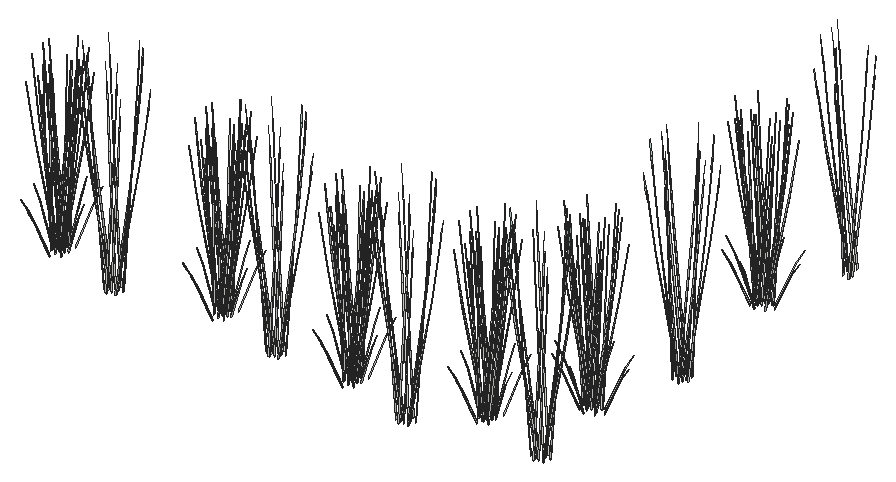
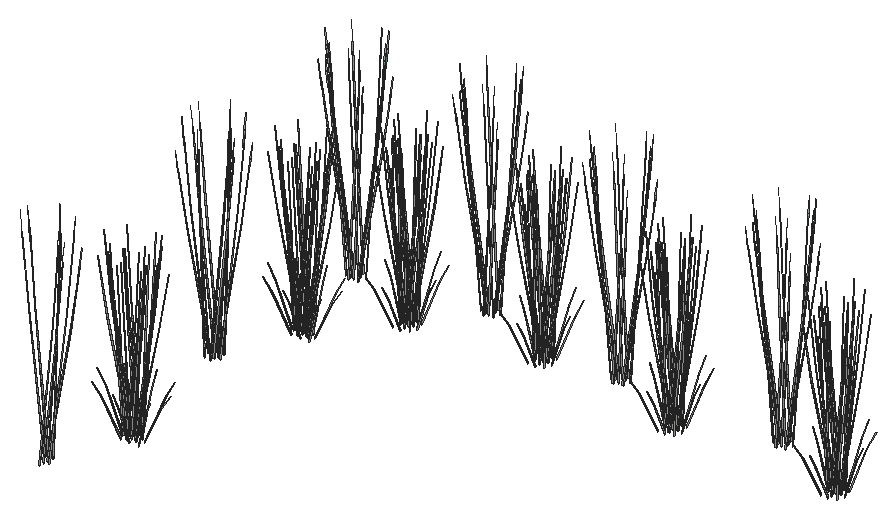
# SketchUp Ruby script. Lengths in inches.
U = 1.inch
M = Sketchup.active_model
def pt(a) = Geom::Point3d.new(a.map { |v| v * U })
def face(e, loops, mat)
  f = e.add_face(loops[0].map { |a| pt(a) })
  loops[1..].each { |l| e.add_face(l.map { |a| pt(a) }).erase! }
  f.material = f.back_material = mat if mat
  f
end
# faces: each face lists its corners as indices into pts; further lists are holes
def faces(e, pts, list, mat = nil) = list.each { |f| face(e, (f[0].is_a?(Array) ? f : [f]).map { |l| l.map { |i| pts[i] } }, mat) }
# xy, xz, yz: faces in a plane at the given z, y or x. An outline is a flat list of corners, or four numbers for a rectangle; further outlines are holes
def ring(l) = l.size == 4 ? [[l[0], l[1]], [l[2], l[1]], [l[2], l[3]], [l[0], l[3]]] : l.each_slice(2).to_a
def flat(e, list, mat, &to3) = list.each { |f| face(e, (f[0].is_a?(Array) ? f : [f]).map { |l| ring(l).map { |u, v| to3.(u, v) } }, mat) }
def xy(e, z, list, mat = nil) = flat(e, list, mat) { |x, y| [x, y, z] }
def xz(e, y, list, mat = nil) = flat(e, list, mat) { |x, z| [x, y, z] }
def yz(e, x, list, mat = nil) = flat(e, list, mat) { |y, z| [x, y, z] }
def lines(e, pts, list) = list.each { |a, b| e.add_line(pt(pts[a]), pt(pts[b])) }
# prism: a flat outline (further loops are holes) pulled along v
def prism(e, loops, v, mat = nil)
  f = face(e, loops, mat); d = Geom::Vector3d.new(v.map { |x| x * U })
  f.pushpull(f.normal.samedirection?(d) ? d.length : -d.length)
end
def box(e, o, s, mat = nil) = prism(e, [[o, [o[0] + s[0], o[1], o[2]], [o[0] + s[0], o[1] + s[1], o[2]], [o[0], o[1] + s[1], o[2]]]], [0, 0, s[2]], mat)
def at(x, y, z, deg = 0) = Geom::Transformation.translation(pt([x, y, z])) * Geom::Transformation.rotation(ORIGIN, Z_AXIS, deg.degrees)
def axes(o, x, y, z) = Geom::Transformation.new([*x, 0, *y, 0, *z, 0, *pt(o).to_a, 1])
def part(name) = M.definitions.add(name)
# library, detail: a bought-in or finely detailed component or shape, given as its bounding box
def library(name, o, s) = part(name).tap { |d| box(d.entities, o, s) }
def detail(e, o, s) = box(e.add_group.entities, o, s)
def put(e, d, t, mat = nil) = e.add_instance(d, t).tap { |i| i.material = mat if mat }
def group(e, t, mat = nil) = e.add_group.tap { |g| g.transformation = t; g.material = mat if mat }.entities
root = M.entities
M.materials.add("LightPink_Translucent").color = [175, 214, 192]
M.materials["LightPink_Translucent"].alpha = 0.75
c1 = part("blade")
p = [[2.15,0.21,22],[0,0.17,0],[0.09,0.45,0],[2.18,0.31,22],[2.29,0.31,22],[0.38,0.45,0],
  [2.48,0.24,33],[2.49,0.24,33],[2.48,0.22,33]]
faces(c1.entities,p,[[0,1,2,3],[4,5,2,3],[6,3,4,7],[8,0,3,6]])
c2 = part("seeds")
p = [[0.3,-0.1,1.38],[-0.01,-0.03,1.59],[-0.01,-0.03,0.03],[0.14,-0.07,-0.07],[0.29,-0.03,3],[0.15,0.01,3.11]]
faces(c2.entities,p,[[0,1,2,3],[1,0,4,5]],"LightPink_Translucent")
c3 = part("blade with seeds")
put(c3.entities,c1,at(0,0,0))
put(c3.entities,c2,axes([2.4,0.25,30.99],[1.5799,-0.05474,1.17369],[-0.12525,1.92788,0.29478],[-0.07173,-0.02425,1.56792]))
c4 = part("blade with seeds\#1")
put(c4.entities,c1,at(0,0,0))
put(root,c3,axes([462.53,231.19,139.17],[-0.19628,-0.45667,-0.6355],[0.5654,-0.16447,-0.16679],[-0.02169,-0.15464,1.40276]))
put(root,c3,axes([461.38,231.125,139.1],[0,-0.44533,-0.45182],[0.53472,0,0],[0,-0.10143,1.43328]))
put(root,c3,axes([462.86,229.81,139.1],[0.44731,-0.22267,-0.45182],[0.26736,0.39927,0],[0.10188,-0.05071,1.43328]))
put(root,c3,axes([463.39,230.72,139.14],[0.32192,-0.33473,-0.56741],[0.39991,0.30352,-0.14892],[0.129,-0.0835,1.25246]))
put(root,c3,axes([462.61,232.04,139.14],[-0.49717,-0.07301,-0.56741],[0.10491,-0.45037,-0.14892],[-0.14837,-0.05457,1.25246]))
put(root,c3,axes([461.96,232.89,139.1],[-0.44731,-0.22267,-0.45182],[0.26736,-0.39927,0],[-0.10188,-0.05071,1.43328]))
put(root,c3,axes([464.93,230.26,139.1],[0.44731,0.22267,-0.45182],[-0.26736,0.39927,0],[0.10188,0.05071,1.43328]))
put(root,c3,axes([464.28,231.11,139.14],[0.49717,0.07301,-0.56741],[-0.10491,0.45037,-0.14892],[0.14837,0.05457,1.25246]))
put(root,c4,axes([445.51,235.44,138.04],[-0.05785,0.02598,1.44662],[-0.33839,-0.1802,-0.221],[-0.00487,-0.18177,0.24641]))
put(root,c3,axes([390.05,236.01,139.08],[-0.19628,-0.45667,-0.6355],[0.5654,-0.16447,-0.16679],[-0.02169,-0.15464,1.40276]))
put(root,c3,axes([428.25,236.01,139.08],[-0.19628,-0.45667,-0.6355],[0.5654,-0.16447,-0.16679],[-0.02169,-0.15464,1.40276]))
put(root,c3,axes([490.26,236.01,139.08],[-0.19628,-0.45667,-0.6355],[0.5654,-0.16447,-0.16679],[-0.02169,-0.15464,1.40276]))
put(root,c3,axes([388.9,235.94,139.01],[0,-0.44533,-0.45182],[0.53472,0,0],[0,-0.10143,1.43328]))
put(root,c3,axes([427.09,235.94,139.01],[0,-0.44533,-0.45182],[0.53472,0,0],[0,-0.10143,1.43328]))
put(root,c3,axes([489.1,235.94,139.01],[0,-0.44533,-0.45182],[0.53472,0,0],[0,-0.10143,1.43328]))
put(root,c3,axes([390.38,234.625,139.01],[0.44731,-0.22267,-0.45182],[0.26736,0.39927,0],[0.10188,-0.05071,1.43328]))
put(root,c3,axes([428.58,234.625,139.01],[0.44731,-0.22267,-0.45182],[0.26736,0.39927,0],[0.10188,-0.05071,1.43328]))
put(root,c3,axes([490.59,234.625,139.01],[0.44731,-0.22267,-0.45182],[0.26736,0.39927,0],[0.10188,-0.05071,1.43328]))
put(root,c3,axes([390.91,235.54,139.04],[0.32192,-0.33473,-0.56741],[0.39991,0.30352,-0.14892],[0.129,-0.0835,1.25246]))
put(root,c3,axes([429.11,235.54,139.04],[0.32192,-0.33473,-0.56741],[0.39991,0.30352,-0.14892],[0.129,-0.0835,1.25246]))
put(root,c3,axes([491.12,235.54,139.04],[0.32192,-0.33473,-0.56741],[0.39991,0.30352,-0.14892],[0.129,-0.0835,1.25246]))
put(root,c4,axes([445.2,237.41,138.5],[0.06247,-0.51713,-0.51151],[0.38535,0.10913,-0.13425],[0.04669,-0.15433,1.12907]))
put(root,c4,axes([447.18,236.76,138.04],[-0.05501,-0.03622,1.44662],[-0.16202,-0.45599,-0.221],[0.08385,-0.13824,0.24641]))
put(root,c3,axes([463.5,232.43,139.14],[-0.32192,0.33473,-0.56741],[-0.39991,-0.30352,-0.14892],[-0.129,0.0835,1.25246]))
put(root,c4,axes([444.47,236.73,138.47],[0.19052,-0.46527,-0.40731],[0.34163,0.2781,0],[0.04339,-0.10597,1.29208]))
put(root,c3,axes([464.03,233.34,139.1],[-0.44731,0.22267,-0.45182],[-0.26736,-0.39927,0],[-0.10188,0.05071,1.43328]))
put(root,c3,axes([465.51,232.03,139.1],[0,0.44533,-0.45182],[-0.53472,0,0],[0,0.10143,1.43328]))
put(root,c4,axes([444.07,236.5,138.04],[-0.03002,0.07441,1.44662],[-0.33536,0.19113,-0.221],[-0.09101,-0.12893,0.24641]))
put(root,c3,axes([464.33,231.97,139.17],[0.17525,0.40774,-0.62983],[-0.50482,0.14685,-0.1653],[0.01937,0.13807,1.39023]))
put(root,c4,axes([444.61,236.86,138.48],[0.33202,-0.11678,-0.25413],[0.09428,0.4638,0.25413],[0.03829,-0.0935,1.14007]))
put(root,c4,axes([444.87,238.33,138.5],[-0.2864,-0.33485,-0.51151],[0.2597,-0.41596,-0.13425],[-0.07144,-0.13418,1.12907]))
put(root,c3,axes([390.13,236.86,139.04],[-0.49717,-0.07301,-0.56741],[0.10491,-0.45037,-0.14892],[-0.14837,-0.05457,1.25246]))
put(root,c3,axes([428.32,236.86,139.04],[-0.49717,-0.07301,-0.56741],[0.10491,-0.45037,-0.14892],[-0.14837,-0.05457,1.25246]))
put(root,c3,axes([490.34,236.86,139.04],[-0.49717,-0.07301,-0.56741],[0.10491,-0.45037,-0.14892],[-0.14837,-0.05457,1.25246]))
put(root,c4,axes([445.32,237.68,138.625],[0.31983,-0.29864,-0.36702],[0.22522,0.45236,0.17663],[0.03957,-0.09664,1.17838]))
put(root,c4,axes([445.98,236.13,138.47],[0.38104,0,-0.40731],[0,0.5562,0],[0.08679,0,1.29208]))
put(root,c3,axes([389.48,237.71,139.01],[-0.44731,-0.22267,-0.45182],[0.26736,-0.39927,0],[-0.10188,-0.05071,1.43328]))
put(root,c3,axes([427.67,237.71,139.01],[-0.44731,-0.22267,-0.45182],[0.26736,-0.39927,0],[-0.10188,-0.05071,1.43328]))
put(root,c3,axes([489.68,237.71,139.01],[-0.44731,-0.22267,-0.45182],[0.26736,-0.39927,0],[-0.10188,-0.05071,1.43328]))
put(root,c3,axes([392.45,235.08,139.01],[0.44731,0.22267,-0.45182],[-0.26736,0.39927,0],[0.10188,0.05071,1.43328]))
put(root,c3,axes([430.64,235.08,139.01],[0.44731,0.22267,-0.45182],[-0.26736,0.39927,0],[0.10188,0.05071,1.43328]))
put(root,c3,axes([492.65,235.08,139.01],[0.44731,0.22267,-0.45182],[-0.26736,0.39927,0],[0.10188,0.05071,1.43328]))
put(root,c4,axes([444.08,238.88,138.47],[-0.19052,-0.46527,-0.40731],[0.34163,-0.2781,0],[-0.04339,-0.10597,1.29208]))
put(root,c4,axes([444.24,238.78,138.48],[0.09428,-0.4638,-0.25413],[0.33202,0.11678,0.25413],[-0.03829,-0.0935,1.14007]))
put(root,c4,axes([445.97,236.37,138.48],[0.23774,0.34702,-0.25413],[-0.23774,0.34702,0.25413],[0.07658,0,1.14007]))
put(root,c4,axes([445.93,237.36,138.53],[0.34888,-0.18229,-0.56778],[0.12565,0.52509,-0.14902],[0.11814,-0.02015,1.25327]))
put(root,c3,axes([391.8,235.93,139.04],[0.49717,0.07301,-0.56741],[-0.10491,0.45037,-0.14892],[0.14837,0.05457,1.25246]))
put(root,c3,axes([429.99,235.93,139.04],[0.49717,0.07301,-0.56741],[-0.10491,0.45037,-0.14892],[0.14837,0.05457,1.25246]))
put(root,c3,axes([492,235.93,139.04],[0.49717,0.07301,-0.56741],[-0.10491,0.45037,-0.14892],[0.14837,0.05457,1.25246]))
put(root,c4,axes([373.03,240.26,137.94],[-0.05785,0.02598,1.44662],[-0.33839,-0.1802,-0.221],[-0.00487,-0.18177,0.24641]))
put(root,c4,axes([411.22,240.26,137.94],[-0.05785,0.02598,1.44662],[-0.33839,-0.1802,-0.221],[-0.00487,-0.18177,0.24641]))
put(root,c4,axes([473.23,240.26,137.94],[-0.05785,0.02598,1.44662],[-0.33839,-0.1802,-0.221],[-0.00487,-0.18177,0.24641]))
put(root,c4,axes([445.83,237.64,138.625],[0.34335,0.2412,-0.36702],[-0.16524,0.50118,0.17663],[0.07915,0,1.17838]))
put(root,c4,axes([447.17,238.89,138.04],[-0.02073,-0.08046,1.44662],[0.11412,-0.48396,-0.221],[0.12863,-0.01415,0.24641]))
put(root,c4,axes([445.37,238.92,138.625],[-0.34335,-0.2412,-0.36702],[0.16524,-0.50118,0.17663],[-0.07915,0,1.17838]))
put(root,c4,axes([443.42,238.54,138.04],[0.01373,0.08339,1.44662],[-0.15453,0.46112,-0.221],[-0.1289,-0.00774,0.24641]))
put(root,c4,axes([372.72,242.23,138.41],[0.06247,-0.51713,-0.51151],[0.38535,0.10913,-0.13425],[0.04669,-0.15433,1.12907]))
put(root,c4,axes([410.91,242.23,138.41],[0.06247,-0.51713,-0.51151],[0.38535,0.10913,-0.13425],[0.04669,-0.15433,1.12907]))
put(root,c4,axes([472.92,242.23,138.41],[0.06247,-0.51713,-0.51151],[0.38535,0.10913,-0.13425],[0.04669,-0.15433,1.12907]))
put(root,c4,axes([374.7,241.58,137.94],[-0.05501,-0.03622,1.44662],[-0.16202,-0.45599,-0.221],[0.08385,-0.13824,0.24641]))
put(root,c4,axes([412.89,241.58,137.94],[-0.05501,-0.03622,1.44662],[-0.16202,-0.45599,-0.221],[0.08385,-0.13824,0.24641]))
put(root,c4,axes([474.9,241.58,137.94],[-0.05501,-0.03622,1.44662],[-0.16202,-0.45599,-0.221],[0.08385,-0.13824,0.24641]))
put(root,c3,axes([391.01,237.25,139.04],[-0.32192,0.33473,-0.56741],[-0.39991,-0.30352,-0.14892],[-0.129,0.0835,1.25246]))
put(root,c3,axes([429.21,237.25,139.04],[-0.32192,0.33473,-0.56741],[-0.39991,-0.30352,-0.14892],[-0.129,0.0835,1.25246]))
put(root,c3,axes([491.22,237.25,139.04],[-0.32192,0.33473,-0.56741],[-0.39991,-0.30352,-0.14892],[-0.129,0.0835,1.25246]))
put(root,c4,axes([371.99,241.55,138.37],[0.19052,-0.46527,-0.40731],[0.34163,0.2781,0],[0.04339,-0.10597,1.29208]))
put(root,c4,axes([410.18,241.55,138.37],[0.19052,-0.46527,-0.40731],[0.34163,0.2781,0],[0.04339,-0.10597,1.29208]))
put(root,c4,axes([472.19,241.55,138.37],[0.19052,-0.46527,-0.40731],[0.34163,0.2781,0],[0.04339,-0.10597,1.29208]))
put(root,c3,axes([391.54,238.16,139.01],[-0.44731,0.22267,-0.45182],[-0.26736,-0.39927,0],[-0.10188,0.05071,1.43328]))
put(root,c3,axes([429.74,238.16,139.01],[-0.44731,0.22267,-0.45182],[-0.26736,-0.39927,0],[-0.10188,0.05071,1.43328]))
put(root,c3,axes([491.75,238.16,139.01],[-0.44731,0.22267,-0.45182],[-0.26736,-0.39927,0],[-0.10188,0.05071,1.43328]))
put(root,c3,axes([393.03,236.84,139.01],[0,0.44533,-0.45182],[-0.53472,0,0],[0,0.10143,1.43328]))
put(root,c3,axes([431.22,236.84,139.01],[0,0.44533,-0.45182],[-0.53472,0,0],[0,0.10143,1.43328]))
put(root,c3,axes([493.24,236.84,139.01],[0,0.44533,-0.45182],[-0.53472,0,0],[0,0.10143,1.43328]))
put(root,c4,axes([371.59,241.31,137.94],[-0.03002,0.07441,1.44662],[-0.33536,0.19113,-0.221],[-0.09101,-0.12893,0.24641]))
put(root,c4,axes([409.79,241.31,137.94],[-0.03002,0.07441,1.44662],[-0.33536,0.19113,-0.221],[-0.09101,-0.12893,0.24641]))
put(root,c4,axes([471.8,241.31,137.94],[-0.03002,0.07441,1.44662],[-0.33536,0.19113,-0.221],[-0.09101,-0.12893,0.24641]))
put(root,c4,axes([445.22,240.19,138.48],[-0.23774,-0.34702,-0.25413],[0.23774,-0.34702,0.25413],[-0.07658,0,1.14007]))
put(root,c4,axes([445.27,239.23,138.53],[-0.39074,0.20416,-0.57289],[-0.14072,-0.5881,-0.15036],[-0.13232,0.02257,1.26456]))
put(root,c4,axes([446.96,237.78,138.48],[-0.09428,0.4638,-0.25413],[-0.33202,-0.11678,0.25413],[0.03829,0.0935,1.14007]))
put(root,c3,axes([391.85,236.78,139.08],[0.17525,0.40774,-0.62983],[-0.50482,0.14685,-0.1653],[0.01937,0.13807,1.39023]))
put(root,c3,axes([430.04,236.78,139.08],[0.17525,0.40774,-0.62983],[-0.50482,0.14685,-0.1653],[0.01937,0.13807,1.39023]))
put(root,c3,axes([492.05,236.78,139.08],[0.17525,0.40774,-0.62983],[-0.50482,0.14685,-0.1653],[0.01937,0.13807,1.39023]))
put(root,c4,axes([447.11,237.68,138.47],[0.19052,0.46527,-0.40731],[-0.34163,0.2781,0],[0.04339,0.10597,1.29208]))
put(root,c4,axes([372.13,241.68,138.38],[0.33202,-0.11678,-0.25413],[0.09428,0.4638,0.25413],[0.03829,-0.0935,1.14007]))
put(root,c4,axes([410.32,241.68,138.38],[0.33202,-0.11678,-0.25413],[0.09428,0.4638,0.25413],[0.03829,-0.0935,1.14007]))
put(root,c4,axes([472.34,241.68,138.38],[0.33202,-0.11678,-0.25413],[0.09428,0.4638,0.25413],[0.03829,-0.0935,1.14007]))
put(root,c4,axes([445.21,240.43,138.47],[-0.38104,0,-0.40731],[0,-0.5562,0],[-0.08679,0,1.29208]))
put(root,c4,axes([372.38,243.15,138.41],[-0.2864,-0.33485,-0.51151],[0.2597,-0.41596,-0.13425],[-0.07144,-0.13418,1.12907]))
put(root,c4,axes([410.58,243.15,138.41],[-0.2864,-0.33485,-0.51151],[0.2597,-0.41596,-0.13425],[-0.07144,-0.13418,1.12907]))
put(root,c4,axes([472.59,243.15,138.41],[-0.2864,-0.33485,-0.51151],[0.2597,-0.41596,-0.13425],[-0.07144,-0.13418,1.12907]))
put(root,c4,axes([446.1,238.24,138.625],[0.02352,0.53984,-0.36702],[-0.39046,0.04882,0.17663],[0.03957,0.09664,1.17838]))
put(root,c4,axes([372.84,242.5,138.53],[0.31983,-0.29864,-0.36702],[0.22522,0.45236,0.17663],[0.03957,-0.09664,1.17838]))
put(root,c4,axes([411.03,242.5,138.53],[0.31983,-0.29864,-0.36702],[0.22522,0.45236,0.17663],[0.03957,-0.09664,1.17838]))
put(root,c4,axes([473.05,242.5,138.53],[0.31983,-0.29864,-0.36702],[0.22522,0.45236,0.17663],[0.03957,-0.09664,1.17838]))
put(root,c4,axes([445.875,238.88,138.625],[-0.31983,0.29864,-0.36702],[-0.22522,-0.45236,0.17663],[-0.03957,0.09664,1.17838]))
put(root,c4,axes([446.33,238.23,138.5],[0.2864,0.33485,-0.51151],[-0.2597,0.41596,-0.13425],[0.07144,0.13418,1.12907]))
put(root,c4,axes([373.5,240.95,138.37],[0.38104,0,-0.40731],[0,0.5562,0],[0.08679,0,1.29208]))
put(root,c4,axes([411.7,240.95,138.37],[0.38104,0,-0.40731],[0,0.5562,0],[0.08679,0,1.29208]))
put(root,c4,axes([473.71,240.95,138.37],[0.38104,0,-0.40731],[0,0.5562,0],[0.08679,0,1.29208]))
put(root,c4,axes([446.58,239.7,138.48],[-0.33202,0.11678,-0.25413],[-0.09428,-0.4638,0.25413],[-0.03829,0.0935,1.14007]))
put(root,c4,axes([371.6,243.7,138.37],[-0.19052,-0.46527,-0.40731],[0.34163,-0.2781,0],[-0.04339,-0.10597,1.29208]))
put(root,c4,axes([409.8,243.7,138.37],[-0.19052,-0.46527,-0.40731],[0.34163,-0.2781,0],[-0.04339,-0.10597,1.29208]))
put(root,c4,axes([471.81,243.7,138.37],[-0.19052,-0.46527,-0.40731],[0.34163,-0.2781,0],[-0.04339,-0.10597,1.29208]))
put(root,c4,axes([371.75,243.59,138.38],[0.09428,-0.4638,-0.25413],[0.33202,0.11678,0.25413],[-0.03829,-0.0935,1.14007]))
put(root,c4,axes([409.95,243.59,138.38],[0.09428,-0.4638,-0.25413],[0.33202,0.11678,0.25413],[-0.03829,-0.0935,1.14007]))
put(root,c4,axes([471.96,243.59,138.38],[0.09428,-0.4638,-0.25413],[0.33202,0.11678,0.25413],[-0.03829,-0.0935,1.14007]))
put(root,c4,axes([373.49,241.1875,138.38],[0.23774,0.34702,-0.25413],[-0.23774,0.34702,0.25413],[0.07658,0,1.14007]))
put(root,c4,axes([411.6875,241.1875,138.38],[0.23774,0.34702,-0.25413],[-0.23774,0.34702,0.25413],[0.07658,0,1.14007]))
put(root,c4,axes([473.7,241.1875,138.38],[0.23774,0.34702,-0.25413],[-0.23774,0.34702,0.25413],[0.07658,0,1.14007]))
put(root,c4,axes([373.45,242.18,138.4375],[0.34888,-0.18229,-0.56778],[0.12565,0.52509,-0.14902],[0.11814,-0.02015,1.25327]))
put(root,c4,axes([411.64,242.18,138.4375],[0.34888,-0.18229,-0.56778],[0.12565,0.52509,-0.14902],[0.11814,-0.02015,1.25327]))
put(root,c4,axes([473.65,242.18,138.4375],[0.34888,-0.18229,-0.56778],[0.12565,0.52509,-0.14902],[0.11814,-0.02015,1.25327]))
put(root,c4,axes([446.73,239.83,138.47],[-0.19052,0.46527,-0.40731],[-0.34163,-0.2781,0],[-0.04339,0.10597,1.29208]))
put(root,c4,axes([443.89,240.03,138.04],[0.0502,0.04815,1.44662],[0.10822,0.48665,-0.221],[-0.09845,0.11756,0.24641]))
put(root,c4,axes([446,239.15,138.5],[-0.06247,0.51713,-0.51151],[-0.38535,-0.10913,-0.13425],[-0.04669,0.15433,1.12907]))
put(root,c4,axes([373.35,242.46,138.53],[0.34335,0.2412,-0.36702],[-0.16524,0.50118,0.17663],[0.07915,0,1.17838]))
put(root,c4,axes([411.54,242.46,138.53],[0.34335,0.2412,-0.36702],[-0.16524,0.50118,0.17663],[0.07915,0,1.17838]))
put(root,c4,axes([473.55,242.46,138.53],[0.34335,0.2412,-0.36702],[-0.16524,0.50118,0.17663],[0.07915,0,1.17838]))
put(root,c4,axes([374.6875,243.71,137.94],[-0.02073,-0.08046,1.44662],[0.11412,-0.48396,-0.221],[0.12863,-0.01415,0.24641]))
put(root,c4,axes([412.88,243.71,137.94],[-0.02073,-0.08046,1.44662],[0.11412,-0.48396,-0.221],[0.12863,-0.01415,0.24641]))
put(root,c4,axes([474.89,243.71,137.94],[-0.02073,-0.08046,1.44662],[0.11412,-0.48396,-0.221],[0.12863,-0.01415,0.24641]))
put(root,c4,axes([447.13,240.95,138.04],[0.03807,-0.06668,1.44662],[0.35272,-0.11307,-0.221],[0.07522,0.14779,0.24641]))
put(root,c4,axes([372.89,243.73,138.53],[-0.34335,-0.2412,-0.36702],[0.16524,-0.50118,0.17663],[-0.07915,0,1.17838]))
put(root,c4,axes([411.08,243.73,138.53],[-0.34335,-0.2412,-0.36702],[0.16524,-0.50118,0.17663],[-0.07915,0,1.17838]))
put(root,c4,axes([473.09,243.73,138.53],[-0.34335,-0.2412,-0.36702],[0.16524,-0.50118,0.17663],[-0.07915,0,1.17838]))
put(root,c4,axes([370.93,243.36,137.94],[0.01373,0.08339,1.44662],[-0.15453,0.46112,-0.221],[-0.1289,-0.00774,0.24641]))
put(root,c4,axes([409.13,243.36,137.94],[0.01373,0.08339,1.44662],[-0.15453,0.46112,-0.221],[-0.1289,-0.00774,0.24641]))
put(root,c4,axes([471.14,243.36,137.94],[0.01373,0.08339,1.44662],[-0.15453,0.46112,-0.221],[-0.1289,-0.00774,0.24641]))
put(root,c4,axes([445.45,240.81,138.04],[0.06005,-0.01261,1.44662],[0.31361,0.25416,-0.221],[-0.01581,0.18053,0.24641]))
put(root,c4,axes([372.74,245.01,138.38],[-0.23774,-0.34702,-0.25413],[0.23774,-0.34702,0.25413],[-0.07658,0,1.14007]))
put(root,c4,axes([410.93,245.01,138.38],[-0.23774,-0.34702,-0.25413],[0.23774,-0.34702,0.25413],[-0.07658,0,1.14007]))
put(root,c4,axes([472.94,245.01,138.38],[-0.23774,-0.34702,-0.25413],[0.23774,-0.34702,0.25413],[-0.07658,0,1.14007]))
put(root,c4,axes([372.78,244.04,138.4375],[-0.39074,0.20416,-0.57289],[-0.14072,-0.5881,-0.15036],[-0.13232,0.02257,1.26456]))
put(root,c4,axes([410.98,244.04,138.4375],[-0.39074,0.20416,-0.57289],[-0.14072,-0.5881,-0.15036],[-0.13232,0.02257,1.26456]))
put(root,c4,axes([472.99,244.04,138.4375],[-0.39074,0.20416,-0.57289],[-0.14072,-0.5881,-0.15036],[-0.13232,0.02257,1.26456]))
put(root,c4,axes([374.48,242.6,138.38],[-0.09428,0.4638,-0.25413],[-0.33202,-0.11678,0.25413],[0.03829,0.0935,1.14007]))
put(root,c4,axes([412.67,242.6,138.38],[-0.09428,0.4638,-0.25413],[-0.33202,-0.11678,0.25413],[0.03829,0.0935,1.14007]))
put(root,c4,axes([474.68,242.6,138.38],[-0.09428,0.4638,-0.25413],[-0.33202,-0.11678,0.25413],[0.03829,0.0935,1.14007]))
put(root,c4,axes([374.63,242.49,138.37],[0.19052,0.46527,-0.40731],[-0.34163,0.2781,0],[0.04339,0.10597,1.29208]))
put(root,c4,axes([412.82,242.49,138.37],[0.19052,0.46527,-0.40731],[-0.34163,0.2781,0],[0.04339,0.10597,1.29208]))
put(root,c4,axes([474.83,242.49,138.37],[0.19052,0.46527,-0.40731],[-0.34163,0.2781,0],[0.04339,0.10597,1.29208]))
put(root,c4,axes([372.73,245.25,138.37],[-0.38104,0,-0.40731],[0,-0.5562,0],[-0.08679,0,1.29208]))
put(root,c4,axes([410.92,245.25,138.37],[-0.38104,0,-0.40731],[0,-0.5562,0],[-0.08679,0,1.29208]))
put(root,c4,axes([472.9375,245.25,138.37],[-0.38104,0,-0.40731],[0,-0.5562,0],[-0.08679,0,1.29208]))
put(root,c4,axes([373.62,243.06,138.53],[0.02352,0.53984,-0.36702],[-0.39046,0.04882,0.17663],[0.03957,0.09664,1.17838]))
put(root,c4,axes([411.82,243.06,138.53],[0.02352,0.53984,-0.36702],[-0.39046,0.04882,0.17663],[0.03957,0.09664,1.17838]))
put(root,c4,axes([473.83,243.06,138.53],[0.02352,0.53984,-0.36702],[-0.39046,0.04882,0.17663],[0.03957,0.09664,1.17838]))
put(root,c4,axes([373.39,243.7,138.53],[-0.31983,0.29864,-0.36702],[-0.22522,-0.45236,0.17663],[-0.03957,0.09664,1.17838]))
put(root,c4,axes([411.59,243.7,138.53],[-0.31983,0.29864,-0.36702],[-0.22522,-0.45236,0.17663],[-0.03957,0.09664,1.17838]))
put(root,c4,axes([473.6,243.7,138.53],[-0.31983,0.29864,-0.36702],[-0.22522,-0.45236,0.17663],[-0.03957,0.09664,1.17838]))
put(root,c4,axes([373.85,243.04,138.41],[0.2864,0.33485,-0.51151],[-0.2597,0.41596,-0.13425],[0.07144,0.13418,1.12907]))
put(root,c4,axes([412.04,243.04,138.41],[0.2864,0.33485,-0.51151],[-0.2597,0.41596,-0.13425],[0.07144,0.13418,1.12907]))
put(root,c4,axes([474.05,243.04,138.41],[0.2864,0.33485,-0.51151],[-0.2597,0.41596,-0.13425],[0.07144,0.13418,1.12907]))
put(root,c4,axes([374.1,244.51,138.38],[-0.33202,0.11678,-0.25413],[-0.09428,-0.4638,0.25413],[-0.03829,0.0935,1.14007]))
put(root,c4,axes([412.3,244.51,138.38],[-0.33202,0.11678,-0.25413],[-0.09428,-0.4638,0.25413],[-0.03829,0.0935,1.14007]))
put(root,c4,axes([474.31,244.51,138.38],[-0.33202,0.11678,-0.25413],[-0.09428,-0.4638,0.25413],[-0.03829,0.0935,1.14007]))
put(root,c4,axes([374.24,244.64,138.37],[-0.19052,0.46527,-0.40731],[-0.34163,-0.2781,0],[-0.04339,0.10597,1.29208]))
put(root,c4,axes([412.4375,244.64,138.37],[-0.19052,0.46527,-0.40731],[-0.34163,-0.2781,0],[-0.04339,0.10597,1.29208]))
put(root,c4,axes([474.45,244.64,138.37],[-0.19052,0.46527,-0.40731],[-0.34163,-0.2781,0],[-0.04339,0.10597,1.29208]))
put(root,c4,axes([371.41,244.85,137.94],[0.0502,0.04815,1.44662],[0.10822,0.48665,-0.221],[-0.09845,0.11756,0.24641]))
put(root,c4,axes([409.6,244.85,137.94],[0.0502,0.04815,1.44662],[0.10822,0.48665,-0.221],[-0.09845,0.11756,0.24641]))
put(root,c4,axes([471.61,244.85,137.94],[0.0502,0.04815,1.44662],[0.10822,0.48665,-0.221],[-0.09845,0.11756,0.24641]))
put(root,c4,axes([373.51,243.96,138.41],[-0.06247,0.51713,-0.51151],[-0.38535,-0.10913,-0.13425],[-0.04669,0.15433,1.12907]))
put(root,c4,axes([411.71,243.96,138.41],[-0.06247,0.51713,-0.51151],[-0.38535,-0.10913,-0.13425],[-0.04669,0.15433,1.12907]))
put(root,c4,axes([473.72,243.96,138.41],[-0.06247,0.51713,-0.51151],[-0.38535,-0.10913,-0.13425],[-0.04669,0.15433,1.12907]))
put(root,c4,axes([374.65,245.76,137.94],[0.03807,-0.06668,1.44662],[0.35272,-0.11307,-0.221],[0.07522,0.14779,0.24641]))
put(root,c4,axes([412.85,245.76,137.94],[0.03807,-0.06668,1.44662],[0.35272,-0.11307,-0.221],[0.07522,0.14779,0.24641]))
put(root,c4,axes([474.86,245.76,137.94],[0.03807,-0.06668,1.44662],[0.35272,-0.11307,-0.221],[0.07522,0.14779,0.24641]))
put(root,c4,axes([372.97,245.63,137.94],[0.06005,-0.01261,1.44662],[0.31361,0.25416,-0.221],[-0.01581,0.18053,0.24641]))
put(root,c4,axes([411.16,245.63,137.94],[0.06005,-0.01261,1.44662],[0.31361,0.25416,-0.221],[-0.01581,0.18053,0.24641]))
put(root,c4,axes([473.18,245.63,137.94],[0.06005,-0.01261,1.44662],[0.31361,0.25416,-0.221],[-0.01581,0.18053,0.24641]))
put(root,c4,axes([486.02,255.62,137.94],[-0.08339,0.01373,1.44662],[-0.46112,-0.15453,-0.221],[0.00774,-0.1289,0.24641]))
put(root,c4,axes([484.53,256.09,137.94],[-0.04815,0.0502,1.44662],[-0.48665,0.10822,-0.221],[-0.11756,-0.09845,0.24641]))
put(root,c4,axes([488.0625,256.28,137.94],[-0.07441,-0.03002,1.44662],[-0.19113,-0.33536,-0.221],[0.12893,-0.09101,0.24641]))
put(root,c4,axes([485.33,257.47,138.4375],[-0.20416,-0.39074,-0.57289],[0.5881,-0.14072,-0.15036],[-0.02257,-0.13232,1.26456]))
put(root,c4,axes([485.67,256.29,138.37],[0.46527,-0.19052,-0.40731],[0.2781,0.34163,0],[0.10597,-0.04339,1.29208]))
put(root,c4,axes([484.13,257.42,138.37],[0,-0.38104,-0.40731],[0.5562,0,0],[0,-0.08679,1.29208]))
put(root,c4,axes([486.22,257.07,138.41],[0.33485,-0.2864,-0.51151],[0.41596,0.2597,-0.13425],[0.13418,-0.07144,1.12907]))
put(root,c4,axes([485.64,257.57,138.53],[0.2412,-0.34335,-0.36702],[0.50118,0.16524,0.17663],[0,-0.07915,1.17838]))
put(root,c4,axes([484.37,257.42,138.38],[0.34702,-0.23774,-0.25413],[0.34702,0.23774,0.25413],[0,-0.07658,1.14007]))
put(root,c4,axes([485.78,256.4375,138.38],[0.4638,0.09428,-0.25413],[-0.11678,0.33202,0.25413],[0.0935,-0.03829,1.14007]))
put(root,c4,axes([485.68,258.08,138.53],[-0.29864,-0.31983,-0.36702],[0.45236,-0.22522,0.17663],[-0.09664,-0.03957,1.17838]))
put(root,c4,axes([485.41,258.2,138.41],[-0.51713,-0.06247,-0.51151],[0.10913,-0.38535,-0.13425],[-0.15433,-0.04669,1.12907]))
put(root,c4,axes([489.11,257.71,137.94],[-0.02598,-0.05785,1.44662],[0.1802,-0.33839,-0.221],[0.18177,-0.00487,0.24641]))
put(root,c4,axes([483.75,257.65,137.94],[0.01261,0.06005,1.44662],[-0.25416,0.31361,-0.221],[-0.18053,-0.01581,0.24641]))
put(root,c4,axes([484.86,258.79,138.38],[-0.11678,-0.33202,-0.25413],[0.4638,-0.09428,0.25413],[-0.0935,-0.03829,1.14007]))
put(root,c4,axes([487.82,256.67,138.37],[0.46527,0.19052,-0.40731],[-0.2781,0.34163,0],[0.10597,0.04339,1.29208]))
put(root,c4,axes([484.73,258.93,138.37],[-0.46527,-0.19052,-0.40731],[0.2781,-0.34163,0],[-0.10597,-0.04339,1.29208]))
put(root,c4,axes([487.69,256.81,138.38],[0.11678,0.33202,-0.25413],[-0.4638,0.09428,0.25413],[0.0935,0.03829,1.14007]))
put(root,c4,axes([487.14,257.4,138.41],[0.51713,0.06247,-0.51151],[-0.10913,0.38535,-0.13425],[0.15433,0.04669,1.12907]))
put(root,c4,axes([486.875,257.52,138.53],[0.29864,0.31983,-0.36702],[-0.45236,0.22522,0.17663],[0.09664,0.03957,1.17838]))
put(root,c4,axes([486.32,258.31,138.53],[-0.53984,0.02352,-0.36702],[-0.04882,-0.39046,0.17663],[-0.09664,0.03957,1.17838]))
put(root,c4,axes([486.77,259.16,138.38],[-0.4638,-0.09428,-0.25413],[0.11678,-0.33202,0.25413],[-0.0935,0.03829,1.14007]))
put(root,c4,axes([488.1875,258.18,138.38],[-0.34702,0.23774,-0.25413],[-0.34702,-0.23774,0.25413],[0,0.07658,1.14007]))
put(root,c4,axes([486.91,258.03,138.53],[-0.2412,0.34335,-0.36702],[-0.50118,-0.16524,0.17663],[0,0.07915,1.17838]))
put(root,c4,axes([486.33,258.53,138.41],[-0.33485,0.2864,-0.51151],[-0.41596,-0.2597,-0.13425],[-0.13418,0.07144,1.12907]))
put(root,c4,axes([488.43,258.1875,138.37],[0,0.38104,-0.40731],[-0.5562,0,0],[0,0.08679,1.29208]))
put(root,c4,axes([486.88,259.3125,138.37],[-0.46527,0.19052,-0.40731],[-0.2781,-0.34163,0],[-0.10597,0.04339,1.29208]))
put(root,c4,axes([487.2,258.13,138.4375],[0.18229,0.34888,-0.56778],[-0.52509,0.12565,-0.14902],[0.02015,0.11814,1.25327]))
put(root,c4,axes([487.8,259.38,137.94],[0.03622,-0.05501,1.44662],[0.45599,-0.16202,-0.221],[0.13824,0.08385,0.24641]))
put(root,c4,axes([483.61,259.34,137.94],[0.06668,0.03807,1.44662],[0.11307,0.35272,-0.221],[-0.14779,0.07522,0.24641]))
put(root,c4,axes([485.67,259.37,137.94],[0.08046,-0.02073,1.44662],[0.48396,0.11412,-0.221],[0.01415,0.12863,0.24641]))
put(root,c3,axes([492.52,274.8125,139.04],[0.07301,-0.49717,-0.56741],[0.45037,0.10491,-0.14892],[0.05457,-0.14837,1.25246]))
put(root,c3,axes([491.66,274.16,139.01],[0.22267,-0.44731,-0.45182],[0.39927,0.26736,0],[0.05071,-0.10188,1.43328]))
put(root,c3,axes([492.125,275.7,139.04],[-0.33473,-0.32192,-0.56741],[0.30352,-0.39991,-0.14892],[-0.0835,-0.129,1.25246]))
put(root,c3,axes([491.21,276.23,139.01],[-0.22267,-0.44731,-0.45182],[0.39927,-0.26736,0],[-0.05071,-0.10188,1.43328]))
put(root,c3,axes([493.43,273.58,139.01],[0.44533,0,-0.45182],[0,0.53472,0],[0.10143,0,1.43328]))
put(root,c3,axes([493.37,274.74,139.08],[0.45667,-0.19628,-0.6355],[0.16447,0.5654,-0.16679],[0.15464,-0.02169,1.40276]))
put(root,c3,axes([492.59,276.53,139.08],[-0.40774,0.17525,-0.62983],[-0.14685,-0.50482,-0.1653],[-0.13807,0.01937,1.39023]))
put(root,c3,axes([492.53,277.71,139.01],[-0.44533,0,-0.45182],[0,-0.53472,0],[-0.10143,0,1.43328]))
put(root,c3,axes([494.75,275.07,139.01],[0.22267,0.44731,-0.45182],[-0.39927,0.26736,0],[0.05071,0.10188,1.43328]))
put(root,c3,axes([493.84,275.6,139.04],[0.33473,0.32192,-0.56741],[-0.30352,0.39991,-0.14892],[0.0835,0.129,1.25246]))
put(root,c3,axes([494.3,277.13,139.01],[-0.22267,0.44731,-0.45182],[-0.39927,-0.26736,0],[-0.05071,0.10188,1.43328]))
put(root,c3,axes([493.45,276.48,139.04],[-0.07301,0.49717,-0.56741],[-0.45037,-0.10491,-0.14892],[-0.05457,0.14837,1.25246]))
put(root,c4,axes([486.02,305.61,137.94],[-0.08339,0.01373,1.44662],[-0.46112,-0.15453,-0.221],[0.00774,-0.1289,0.24641]))
put(root,c4,axes([484.53,306.08,137.94],[-0.04815,0.0502,1.44662],[-0.48665,0.10822,-0.221],[-0.11756,-0.09845,0.24641]))
put(root,c4,axes([488.0625,306.26,137.94],[-0.07441,-0.03002,1.44662],[-0.19113,-0.33536,-0.221],[0.12893,-0.09101,0.24641]))
put(root,c4,axes([485.33,307.46,138.4375],[-0.20416,-0.39074,-0.57289],[0.5881,-0.14072,-0.15036],[-0.02257,-0.13232,1.26456]))
put(root,c4,axes([485.67,306.28,138.37],[0.46527,-0.19052,-0.40731],[0.2781,0.34163,0],[0.10597,-0.04339,1.29208]))
put(root,c4,axes([484.13,307.4,138.37],[0,-0.38104,-0.40731],[0.5562,0,0],[0,-0.08679,1.29208]))
put(root,c4,axes([486.22,307.06,138.41],[0.33485,-0.2864,-0.51151],[0.41596,0.2597,-0.13425],[0.13418,-0.07144,1.12907]))
put(root,c4,axes([485.64,307.56,138.53],[0.2412,-0.34335,-0.36702],[0.50118,0.16524,0.17663],[0,-0.07915,1.17838]))
put(root,c4,axes([484.37,307.41,138.38],[0.34702,-0.23774,-0.25413],[0.34702,0.23774,0.25413],[0,-0.07658,1.14007]))
put(root,c4,axes([485.78,306.43,138.38],[0.4638,0.09428,-0.25413],[-0.11678,0.33202,0.25413],[0.0935,-0.03829,1.14007]))
put(root,c4,axes([485.68,308.0625,138.53],[-0.29864,-0.31983,-0.36702],[0.45236,-0.22522,0.17663],[-0.09664,-0.03957,1.17838]))
put(root,c4,axes([485.41,308.1875,138.41],[-0.51713,-0.06247,-0.51151],[0.10913,-0.38535,-0.13425],[-0.15433,-0.04669,1.12907]))
put(root,c4,axes([489.11,307.7,137.94],[-0.02598,-0.05785,1.44662],[0.1802,-0.33839,-0.221],[0.18177,-0.00487,0.24641]))
put(root,c4,axes([483.75,307.64,137.94],[0.01261,0.06005,1.44662],[-0.25416,0.31361,-0.221],[-0.18053,-0.01581,0.24641]))
put(root,c4,axes([484.86,308.77,138.38],[-0.11678,-0.33202,-0.25413],[0.4638,-0.09428,0.25413],[-0.0935,-0.03829,1.14007]))
put(root,c4,axes([487.82,306.66,138.37],[0.46527,0.19052,-0.40731],[-0.2781,0.34163,0],[0.10597,0.04339,1.29208]))
put(root,c4,axes([484.73,308.92,138.37],[-0.46527,-0.19052,-0.40731],[0.2781,-0.34163,0],[-0.10597,-0.04339,1.29208]))
put(root,c4,axes([487.69,306.8,138.38],[0.11678,0.33202,-0.25413],[-0.4638,0.09428,0.25413],[0.0935,0.03829,1.14007]))
put(root,c4,axes([487.14,307.39,138.41],[0.51713,0.06247,-0.51151],[-0.10913,0.38535,-0.13425],[0.15433,0.04669,1.12907]))
put(root,c4,axes([486.875,307.51,138.53],[0.29864,0.31983,-0.36702],[-0.45236,0.22522,0.17663],[0.09664,0.03957,1.17838]))
put(root,c4,axes([486.32,308.29,138.53],[-0.53984,0.02352,-0.36702],[-0.04882,-0.39046,0.17663],[-0.09664,0.03957,1.17838]))
put(root,c4,axes([486.77,309.15,138.38],[-0.4638,-0.09428,-0.25413],[0.11678,-0.33202,0.25413],[-0.0935,0.03829,1.14007]))
put(root,c4,axes([488.1875,308.17,138.38],[-0.34702,0.23774,-0.25413],[-0.34702,-0.23774,0.25413],[0,0.07658,1.14007]))
put(root,c4,axes([486.91,308.02,138.53],[-0.2412,0.34335,-0.36702],[-0.50118,-0.16524,0.17663],[0,0.07915,1.17838]))
put(root,c4,axes([486.33,308.52,138.41],[-0.33485,0.2864,-0.51151],[-0.41596,-0.2597,-0.13425],[-0.13418,0.07144,1.12907]))
put(root,c4,axes([488.43,308.17,138.37],[0,0.38104,-0.40731],[-0.5562,0,0],[0,0.08679,1.29208]))
put(root,c4,axes([486.88,309.3,138.37],[-0.46527,0.19052,-0.40731],[-0.2781,-0.34163,0],[-0.10597,0.04339,1.29208]))
put(root,c4,axes([487.2,308.12,138.4375],[0.18229,0.34888,-0.56778],[-0.52509,0.12565,-0.14902],[0.02015,0.11814,1.25327]))
put(root,c4,axes([487.8,309.37,137.94],[0.03622,-0.05501,1.44662],[0.45599,-0.16202,-0.221],[0.13824,0.08385,0.24641]))
put(root,c4,axes([483.61,309.32,137.94],[0.06668,0.03807,1.44662],[0.11307,0.35272,-0.221],[-0.14779,0.07522,0.24641]))
put(root,c4,axes([485.67,309.36,137.94],[0.08046,-0.02073,1.44662],[0.48396,0.11412,-0.221],[0.01415,0.12863,0.24641]))
put(root,c3,axes([492.52,324.8,139.04],[0.07301,-0.49717,-0.56741],[0.45037,0.10491,-0.14892],[0.05457,-0.14837,1.25246]))
put(root,c3,axes([491.66,324.15,139.01],[0.22267,-0.44731,-0.45182],[0.39927,0.26736,0],[0.05071,-0.10188,1.43328]))
put(root,c3,axes([492.125,325.6875,139.04],[-0.33473,-0.32192,-0.56741],[0.30352,-0.39991,-0.14892],[-0.0835,-0.129,1.25246]))
put(root,c3,axes([491.21,326.22,139.01],[-0.22267,-0.44731,-0.45182],[0.39927,-0.26736,0],[-0.05071,-0.10188,1.43328]))
put(root,c3,axes([493.43,323.57,139.01],[0.44533,0,-0.45182],[0,0.53472,0],[0.10143,0,1.43328]))
put(root,c3,axes([493.37,324.73,139.08],[0.45667,-0.19628,-0.6355],[0.16447,0.5654,-0.16679],[0.15464,-0.02169,1.40276]))
put(root,c3,axes([492.59,326.52,139.08],[-0.40774,0.17525,-0.62983],[-0.14685,-0.50482,-0.1653],[-0.13807,0.01937,1.39023]))
put(root,c3,axes([492.53,327.7,139.01],[-0.44533,0,-0.45182],[0,-0.53472,0],[-0.10143,0,1.43328]))
